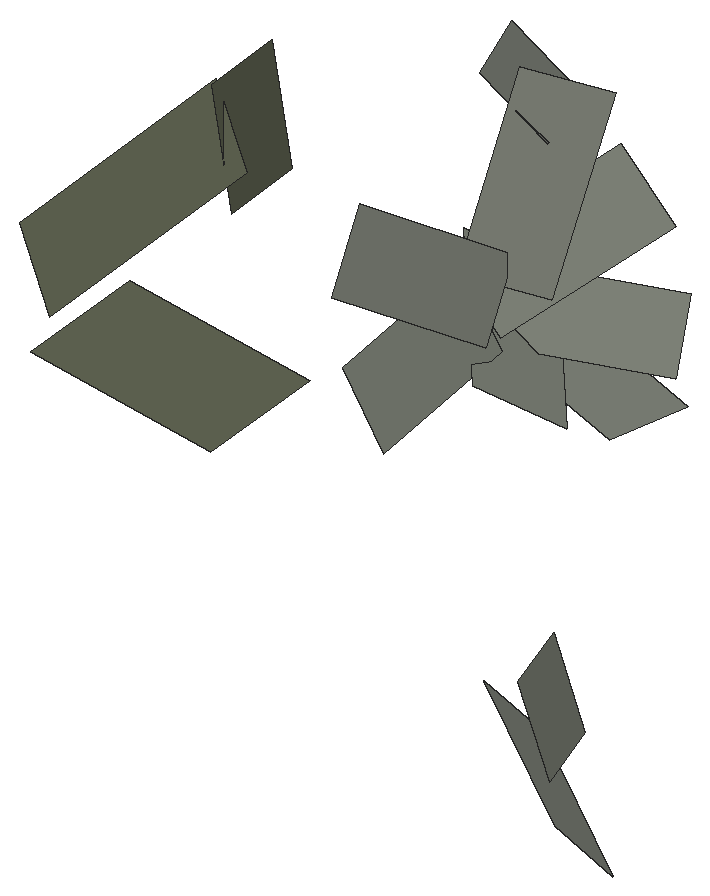
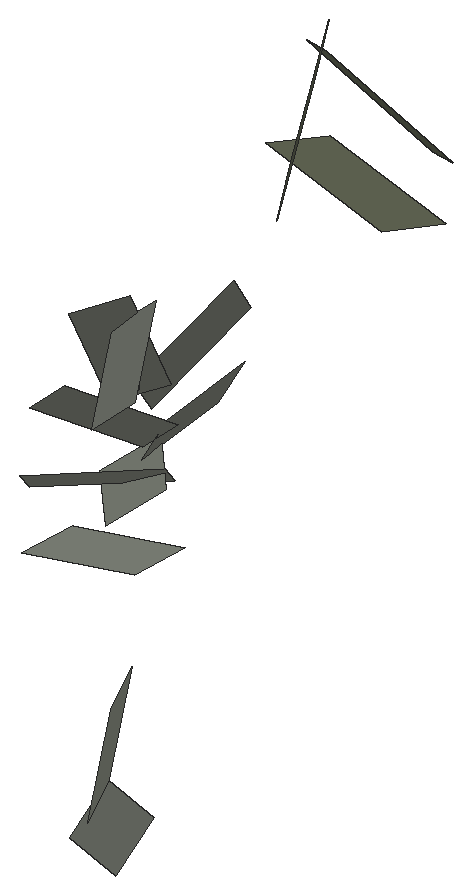
# SketchUp Ruby script. Lengths in inches.
U = 1.inch
M = Sketchup.active_model
def pt(a) = Geom::Point3d.new(a.map { |v| v * U })
def face(e, loops, mat)
  f = e.add_face(loops[0].map { |a| pt(a) })
  loops[1..].each { |l| e.add_face(l.map { |a| pt(a) }).erase! }
  f.material = f.back_material = mat if mat
  f
end
# faces: each face lists its corners as indices into pts; further lists are holes
def faces(e, pts, list, mat = nil) = list.each { |f| face(e, (f[0].is_a?(Array) ? f : [f]).map { |l| l.map { |i| pts[i] } }, mat) }
# xy, xz, yz: faces in a plane at the given z, y or x. An outline is a flat list of corners, or four numbers for a rectangle; further outlines are holes
def ring(l) = l.size == 4 ? [[l[0], l[1]], [l[2], l[1]], [l[2], l[3]], [l[0], l[3]]] : l.each_slice(2).to_a
def flat(e, list, mat, &to3) = list.each { |f| face(e, (f[0].is_a?(Array) ? f : [f]).map { |l| ring(l).map { |u, v| to3.(u, v) } }, mat) }
def xy(e, z, list, mat = nil) = flat(e, list, mat) { |x, y| [x, y, z] }
def xz(e, y, list, mat = nil) = flat(e, list, mat) { |x, z| [x, y, z] }
def yz(e, x, list, mat = nil) = flat(e, list, mat) { |y, z| [x, y, z] }
def lines(e, pts, list) = list.each { |a, b| e.add_line(pt(pts[a]), pt(pts[b])) }
# prism: a flat outline (further loops are holes) pulled along v
def prism(e, loops, v, mat = nil)
  f = face(e, loops, mat); d = Geom::Vector3d.new(v.map { |x| x * U })
  f.pushpull(f.normal.samedirection?(d) ? d.length : -d.length)
end
def box(e, o, s, mat = nil) = prism(e, [[o, [o[0] + s[0], o[1], o[2]], [o[0] + s[0], o[1] + s[1], o[2]], [o[0], o[1] + s[1], o[2]]]], [0, 0, s[2]], mat)
def at(x, y, z, deg = 0) = Geom::Transformation.translation(pt([x, y, z])) * Geom::Transformation.rotation(ORIGIN, Z_AXIS, deg.degrees)
def axes(o, x, y, z) = Geom::Transformation.new([*x, 0, *y, 0, *z, 0, *pt(o).to_a, 1])
def part(name) = M.definitions.add(name)
# library, detail: a bought-in or finely detailed component or shape, given as its bounding box
def library(name, o, s) = part(name).tap { |d| box(d.entities, o, s) }
def detail(e, o, s) = box(e.add_group.entities, o, s)
def put(e, d, t, mat = nil) = e.add_instance(d, t).tap { |i| i.material = mat if mat }
def group(e, t, mat = nil) = e.add_group.tap { |g| g.transformation = t; g.material = mat if mat }.entities
root = M.entities
M.materials.add("viburnumblaasdfas0df1w06d").color = [98, 102, 84]
M.materials.add("viburnumbladsadfasdfad0w122").color = [125, 129, 119]
c1 = part("Component\#315")
p = [[0.25,0,0],[2.05,0.01,0.35],[1.81,4.2,1.66],[0,4.19,1.3125]]
faces(c1.entities,p,[[0,1,2,3]],"viburnumbladsadfasdfad0w122")
c2 = part("viburnumblad2")
put(c2.entities,c1,axes([-19.23,-4.49,-32.18],[83.35428,0,0],[0,79.38502,0],[0,0,83.35428]))
c3 = part("Component\#314")
p = [[0.14,0,0],[2.58,0.05,0.25],[2.44,5.11,2.64],[0,5.05,2.39]]
faces(c3.entities,p,[[0,1,2,3]],"viburnumblaasdfas0df1w06d")
c4 = part("viburnumblad1\#2")
put(c4.entities,c3,axes([-37.25,6.23,19.31],[75.98784,0,0],[0,65.50676,0],[0,0,75.98784]))
put(root,c2,axes([1243.64,210.84,25.04],[-0.00974,-0.00261,0.006],[0.00353,-0.01123,0.00072],[0.00551,0.00254,0.00899]))
put(root,c2,axes([1242.62,211.21,11.1875],[-0.00427,-0.00859,0.00811],[0.00683,-0.00794,-0.00482],[0.00917,0.00302,0.00803]))
put(root,c2,axes([1242.1,210.8,21.01],[-0.00288,-0.01252,-0.00147],[0.01138,-0.00177,-0.00721],[0.00645,-0.00276,0.01087]))
put(root,c4,axes([1241.98,196.5625,27.34],[0.00886,-0.00621,-0.00526],[0.00932,0.00889,0.00498],[0.00073,-0.00681,0.00878]))
put(root,c2,axes([1243.73,210.03,21.68],[-0.00909,-0.00791,0.00471],[0.00591,-0.01009,-0.00553],[0.00706,-0.00173,0.0107]))
put(root,c2,axes([1244.2,210.48,12.02],[-0.00745,0.00026,0.01011],[0.00262,-0.01208,0.00224],[0.00977,0.00344,0.00711]))
put(root,c2,axes([1245.08,206.73,21.75],[-0.00733,-0.00034,0.00907],[-0.00172,-0.01154,-0.00184],[0.00876,-0.00225,0.00608]))
put(root,c4,axes([1243.625,201.91,27.5],[-0.00543,0.00233,0.01137],[0.00034,-0.01453,0.00314],[0.0116,0.00141,0.00526]))
put(root,c2,axes([1245.71,205.47,22.61],[-0.00322,0.00766,0.00823],[-0.00606,-0.00853,0.00527],[0.00929,-0.00262,0.00521]))
put(root,c2,axes([1243.27,207.96,22.62],[0.0022,-0.00655,-0.00816],[0.00813,0.00764,-0.00386],[0.00785,-0.0054,0.00541]))
put(root,c2,axes([1243.77,206.72,23.34],[0.00733,0.00034,-0.00907],[0.00348,0.00978,0.00299],[0.00808,-0.00497,0.00546]))
put(root,c4,axes([1242.58,198.38,25.6875],[-0.00299,-0.01191,-0.00429],[0.01424,-0.00187,-0.0047],[0.00288,-0.00486,0.01046]))
put(root,c2,axes([1244.86,205.66,23.79],[0.00715,0.00814,-0.0046],[-0.00216,0.00716,0.00888],[0.00881,-0.00455,0.00477]))
